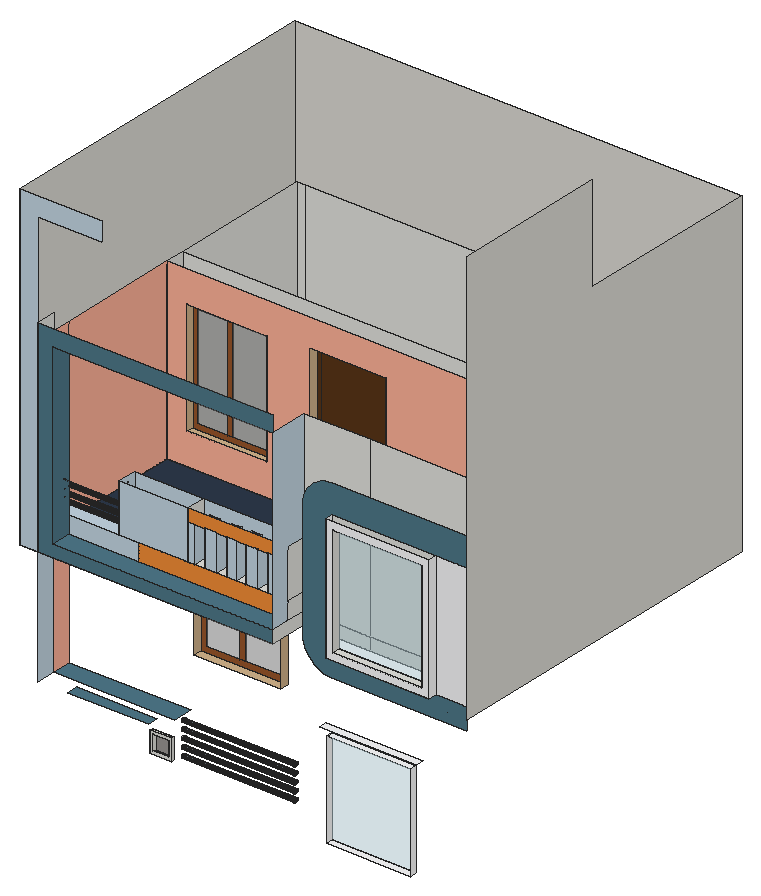
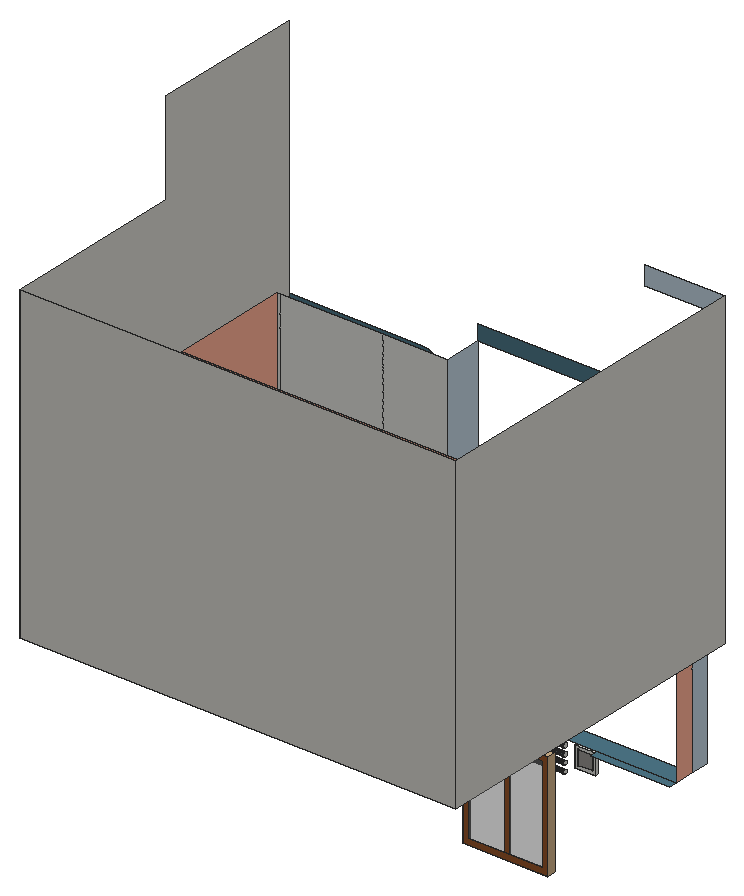
# SketchUp Ruby script. Lengths in inches.
U = 1.inch
M = Sketchup.active_model
def pt(a) = Geom::Point3d.new(a.map { |v| v * U })
def face(e, loops, mat)
  f = e.add_face(loops[0].map { |a| pt(a) })
  loops[1..].each { |l| e.add_face(l.map { |a| pt(a) }).erase! }
  f.material = f.back_material = mat if mat
  f
end
# faces: each face lists its corners as indices into pts; further lists are holes
def faces(e, pts, list, mat = nil) = list.each { |f| face(e, (f[0].is_a?(Array) ? f : [f]).map { |l| l.map { |i| pts[i] } }, mat) }
# xy, xz, yz: faces in a plane at the given z, y or x. An outline is a flat list of corners, or four numbers for a rectangle; further outlines are holes
def ring(l) = l.size == 4 ? [[l[0], l[1]], [l[2], l[1]], [l[2], l[3]], [l[0], l[3]]] : l.each_slice(2).to_a
def flat(e, list, mat, &to3) = list.each { |f| face(e, (f[0].is_a?(Array) ? f : [f]).map { |l| ring(l).map { |u, v| to3.(u, v) } }, mat) }
def xy(e, z, list, mat = nil) = flat(e, list, mat) { |x, y| [x, y, z] }
def xz(e, y, list, mat = nil) = flat(e, list, mat) { |x, z| [x, y, z] }
def yz(e, x, list, mat = nil) = flat(e, list, mat) { |y, z| [x, y, z] }
def lines(e, pts, list) = list.each { |a, b| e.add_line(pt(pts[a]), pt(pts[b])) }
# prism: a flat outline (further loops are holes) pulled along v
def prism(e, loops, v, mat = nil)
  f = face(e, loops, mat); d = Geom::Vector3d.new(v.map { |x| x * U })
  f.pushpull(f.normal.samedirection?(d) ? d.length : -d.length)
end
def box(e, o, s, mat = nil) = prism(e, [[o, [o[0] + s[0], o[1], o[2]], [o[0] + s[0], o[1] + s[1], o[2]], [o[0], o[1] + s[1], o[2]]]], [0, 0, s[2]], mat)
def at(x, y, z, deg = 0) = Geom::Transformation.translation(pt([x, y, z])) * Geom::Transformation.rotation(ORIGIN, Z_AXIS, deg.degrees)
def axes(o, x, y, z) = Geom::Transformation.new([*x, 0, *y, 0, *z, 0, *pt(o).to_a, 1])
def part(name) = M.definitions.add(name)
# library, detail: a bought-in or finely detailed component or shape, given as its bounding box
def library(name, o, s) = part(name).tap { |d| box(d.entities, o, s) }
def detail(e, o, s) = box(e.add_group.entities, o, s)
def put(e, d, t, mat = nil) = e.add_instance(d, t).tap { |i| i.material = mat if mat }
def group(e, t, mat = nil) = e.add_group.tap { |g| g.transformation = t; g.material = mat if mat }.entities
root = M.entities
M.materials.add("[0035_Tan]").color = [210, 180, 140]
M.materials.add("[0096_SkyBlue]").color = [79, 120, 137]
M.materials.add("[Blinds Vertical Pattern]").color = [247, 247, 249]
M.materials.add("[Cladding Siding Tan]").color = [242, 141, 55]
M.materials.add("[Color B02]").color = [255, 178, 153]
M.materials.add("[Concrete Aggregate Smoke]").color = [154, 150, 148]
M.materials.add("[Formica Speckled Grey]").color = [94, 105, 111]
M.materials.add("[Leather Blue]").color = [45, 57, 74]
M.materials.add("[Quartz Light Grey]").color = [251, 251, 252]
M.materials.add("[Terrazzo Light Blue]").color = [196, 214, 227]
M.materials.add("[Terrazzo Tile Light]").color = [219, 217, 210]
M.materials.add("[Translucent Glass Gray]1").color = [128, 128, 128]
M.materials["[Translucent Glass Gray]1"].alpha = 0.5
M.materials.add("[Translucent Glass Safety]").color = [204, 235, 244]
M.materials["[Translucent Glass Safety]"].alpha = 0.5
M.materials.add("[Wood Cherry Original]1").color = [152, 86, 42]
M.materials.add("[Wood Floor Parquet]").color = [89, 54, 24]
xy(root,174.45,[[254.96,158.43,308.4,162.87]],"[Quartz Light Grey]")
xy(root,175.17,[[85.49,265.26,140.61,270.89]],"[0035_Tan]")
xy(root,175.61,[[131.3,173.37,144.73,175.06]])
xy(root,177.5,[[133.18,173.37,142.85,175.06]])
xy(root,187.17,[[133.18,173.37,142.85,175.06]])
xy(root,189.05,[[131.3,173.37,144.73,175.06]])
xy(root,190.75,[[77.92,175.06,129.11,181.62]],"[0096_SkyBlue]")
xy(root,199,[[68.53,175.06,145.53,187.5]],"[0096_SkyBlue]")
xy(root,235.33,[[254.96,158.43,308.4,162.87]],"[Quartz Light Grey]")
xy(root,239.3,[[250.99,158.43,312.37,162.87]],"[Quartz Light Grey]")
xy(root,244.54,[[85.49,265.26,140.61,270.89]],"[0035_Tan]")
xy(root,252.25,[[159.93,265.26,209.68,271.64]],"[0035_Tan]")
xy(root,272.8125,[[57.16,162.87,68.53,175.06],[68.53,265.26,328.05,277.89],[68.53,277.89,73.72,368.29],[73.72,277.89,328.05,368.29]])
xy(root,272.8125,[[68.53,162.87,68.53,265.26,328.05,265.26,328.05,187.5,217.34,187.5,217.34,162.87]],"[Color B02]")
xy(root,280.09,[[254.93,157.81,320.55,162.87]])
xy(root,280.8125,[[68.53,175.18,217.34,187.5],[68.53,265.26,68.53,277.89,328.05,277.89,328.05,265.26,207.48,265.26,207.48,270.7,158.92,270.7,158.92,265.26],[68.53,277.89,328.05,368.29]])
xy(root,280.8125,[[158.92,265.26,207.48,270.7]],"[0035_Tan]")
xy(root,280.8125,[[78.16,162.87,217.34,175.18]],"[0096_SkyBlue]")
xy(root,280.8125,[[68.53,187.5,328.05,265.26]],"[Leather Blue]")
xy(root,284.73,[[259.5625,157.81,315.92,162.87]])
xy(root,291.5625,[[110.1875,175.18,153.69,187.5],[153.69,175.18,158.09,187.5],[158.09,175.18,164.38,187.5],[164.38,175.18,171.84,187.5],[171.84,175.18,178.13,187.5],
  [178.13,175.18,184.46,187.5],[184.46,175.18,190.75,187.5],[190.75,175.18,198.34,187.5],[198.34,175.18,204.63,187.5],[204.63,175.18,217.34,187.5]])
xy(root,291.5625,[[68.53,175.18,110.1875,187.5]],"[Terrazzo Light Blue]")
xy(root,301.03,[[81.24,265.26,131.93,269.39]],"[0035_Tan]")
xz(root,157.81,[[[254.93,280.09,320.55,358.97],[259.5625,284.73,315.92,354.33]]],"[Quartz Light Grey]")
xz(root,162.87,[[[254.93,280.09,320.55,358.97],[259.5625,284.73,315.92,354.33]]])
xz(root,162.87,[[254.82,266.71,340.49,266.71,340.49,280.09,254.93,280.09,254.93,358.97,340.49,358.97,340.49,377.3,254.93,377.3,252.54,377.14,250.18,376.67,247.91,375.9,245.76,374.84,243.77,373.51,241.97,371.93,240.38,370.125,239.05,368.13,237.99,365.98,237.22,363.71,236.75,361.36,236.6,358.97,236.6,284.93,236.75,282.55,237.22,280.21,237.98,277.95,239.04,275.82,240.36,273.84,241.93,272.04,243.72,270.47,245.71,269.15,247.84,268.09,250.1,267.33,252.4375,266.86],[68.53,272.8125,217.34,272.8125,217.34,280.8125,78.16,280.8125,78.16,392.8125,217.34,392.8125,217.34,403.0625,68.53,403.0625]],"[0096_SkyBlue]")
xz(root,162.87,[[320.55,280.09,340.49,358.97]],"[Blinds Vertical Pattern]")
xz(root,162.87,[[57.16,272.8125,68.53,272.8125,68.53,463,109.08,463,109.08,475.0625,57.16,475.0625]],"[Terrazzo Light Blue]")
xz(root,162.87,[[254.96,174.45,308.4,235.33],[259.5625,284.73,315.92,354.33]],"[Translucent Glass Safety]")
xz(root,173.37,[[[131.3,175.61,144.73,189.05],[133.18,177.5,142.85,187.17]]])
xz(root,175.06,[[[131.3,175.61,144.73,189.05],[133.18,177.5,142.85,187.17]]])
xz(root,175.06,[[133.18,177.5,142.85,187.17]],"[Concrete Aggregate Smoke]")
xz(root,175.18,[[68.53,280.8125,78.16,291.5625],[68.53,291.5625,78.16,392.8125]])
xz(root,175.18,[[122.76,280.8125,217.34,291.5625],[210.19,291.5625,217.34,291.5625,217.34,322.125,153.69,322.125,153.69,314.29,210.19,314.29]],"[Cladding Siding Tan]")
xz(root,175.18,[[78.16,280.8125,122.76,291.5625],[110.1875,291.5625,153.69,322.125],[153.69,291.5625,158.09,314.29],[164.38,291.5625,171.84,314.29],[178.13,291.5625,184.46,314.29],
  [190.75,291.5625,198.34,314.29],[204.63,291.5625,210.19,314.29]],"[Terrazzo Light Blue]")
xz(root,187.5,[[217.34,272.8125,259.37,280.8125],[259.37,272.8125,326.14,280.8125],[326.14,272.8125,328.05,280.8125],[217.34,280.8125,259.37,392.8125],[259.37,280.8125,326.14,392.8125],
  [326.14,280.8125,328.05,392.8125]])
xz(root,187.5,[[68.53,280.8125,217.34,291.5625],[110.1875,291.5625,153.69,322.125],[153.69,291.5625,153.69,322.125,217.34,322.125,217.34,291.5625,204.63,291.5625,204.63,314.29,198.34,314.29,198.34,291.5625,190.75,291.5625,190.75,314.29,184.46,314.29,184.46,291.5625,178.13,291.5625,178.13,314.29,171.84,314.29,171.84,291.5625,164.38,291.5625,164.38,314.29,158.09,314.29,158.09,291.5625]],"[Terrazzo Light Blue]")
xz(root,265.26,[[68.53,272.8125,328.05,280.8125]])
xz(root,265.26,[[[68.53,280.8125,158.92,280.8125,158.92,375.1875,207.48,375.1875,207.48,280.8125,328.05,280.8125,328.05,392.8125,68.53,392.8125],[81.24,301.03,131.93,372.97]]],"[Color B02]")
xz(root,269.39,[[84.54,304.33,103.99,369.67],[106.67,304.33,128.62,369.67]],"[Translucent Glass Gray]1")
xz(root,269.39,[[[81.24,301.03,131.93,372.97],[84.54,304.33,128.62,369.67]],[103.99,304.33,106.67,369.67]],"[Wood Cherry Original]1")
xz(root,270.7,[[[158.92,280.8125,207.48,375.1875],[162.2,284.1,204.19,371.9]],[162.2,284.1,204.19,371.9]],"[Wood Floor Parquet]")
xz(root,270.89,[[89.04,178.72,110.22,241],[113.79,178.72,137.07,241]],"[Translucent Glass Gray]1")
xz(root,270.89,[[[85.49,175.17,140.61,244.54],[89.04,178.72,137.07,241]],[110.22,178.72,113.79,241]],"[Wood Cherry Original]1")
xz(root,277.89,[[68.53,272.8125,328.05,280.8125],[68.53,280.8125,328.05,392.8125]])
xz(root,368.29,[[68.53,272.8125,73.72,280.8125],[73.72,272.8125,328.05,280.8125],[68.53,280.8125,73.72,392.8125],[73.72,280.8125,328.05,392.8125]])
xz(root,380.73,[[57.16,272.8125,340.49,475.0625]],"[Terrazzo Tile Light]")
yz(root,57.16,[[162.87,272.8125,380.73,475.0625]],"[Terrazzo Tile Light]")
yz(root,68.53,[[162.87,272.8125,187.5,280.8125],[187.5,272.8125,265.26,280.8125],[265.26,272.8125,277.89,280.8125],[277.89,272.8125,368.29,280.8125],[162.87,280.8125,175.18,403.0625],
  [175.18,280.8125,187.5,291.5625],[265.26,280.8125,277.89,392.8125],[277.89,280.8125,368.29,392.8125]])
yz(root,68.53,[[175.06,199,187.5,272.8125],[187.5,280.8125,265.26,392.8125],[[175.18,291.5625,187.5,392.8125],[181.95,297.93,181.66,297.97,181.39,298.08,181.16,298.26,180.98,298.5,180.86,298.77,180.83,299.06,180.86,299.35,180.98,299.62,181.16,299.85,181.39,300.03,181.66,300.15,181.95,300.18,182.24,300.15,182.51,300.03,182.75,299.85,182.93,299.62,183.04,299.35,183.08,299.06,183.04,298.77,182.93,298.5,182.75,298.26,182.51,298.08,182.24,297.97],[181.95,293.37,181.66,293.41,181.39,293.52,181.16,293.7,180.98,293.93,180.86,294.21,180.83,294.5,180.86,294.79,180.98,295.06,181.16,295.29,181.39,295.47,181.66,295.58,181.95,295.62,182.24,295.58,182.51,295.47,182.75,295.29,182.93,295.06,183.04,294.79,183.08,294.5,183.04,294.21,182.93,293.93,182.75,293.7,182.51,293.52,182.24,293.41],[181.95,303.25,181.66,303.28,181.39,303.4,181.16,303.58,180.98,303.81,180.86,304.08,180.83,304.37,180.86,304.66,180.98,304.93,181.16,305.17,181.39,305.35,181.66,305.46,181.95,305.5,182.24,305.46,182.51,305.35,182.75,305.17,182.93,304.93,183.04,304.66,183.08,304.37,183.04,304.08,182.93,303.81,182.75,303.58,182.51,303.4,182.24,303.28],[181.95,308.5,181.66,308.53,181.39,308.65,181.16,308.83,180.98,309.06,180.86,309.33,180.83,309.62,180.86,309.91,180.98,310.18,181.16,310.42,181.39,310.6,181.66,310.71,181.95,310.75,182.24,310.71,182.51,310.6,182.75,310.42,182.93,310.18,183.04,309.91,183.08,309.62,183.04,309.33,182.93,309.06,182.75,308.83,182.51,308.65,182.24,308.53],[181.95,313,181.66,313.03,181.39,313.15,181.16,313.33,180.98,313.56,180.86,313.83,180.83,314.12,180.86,314.41,180.98,314.68,181.16,314.92,181.39,315.1,181.66,315.21,181.95,315.25,182.24,315.21,182.51,315.1,182.75,314.92,182.93,314.68,183.04,314.41,183.08,314.12,183.04,313.83,182.93,313.56,182.75,313.33,182.51,313.15,182.24,313.03],[181.95,317.18,181.66,317.22,181.39,317.33,181.16,317.51,180.98,317.75,180.86,318.02,180.83,318.31,180.86,318.6,180.98,318.87,181.16,319.1,181.39,319.28,181.66,319.4,181.95,319.43,182.24,319.4,182.51,319.28,182.75,319.1,182.93,318.87,183.04,318.6,183.08,318.31,183.04,318.02,182.93,317.75,182.75,317.51,182.51,317.33,182.24,317.22]]],"[Color B02]")
yz(root,68.53,[[162.87,199,175.06,272.8125]],"[Terrazzo Light Blue]")
yz(root,78.16,[[162.87,280.8125,175.18,392.8125]],"[0096_SkyBlue]")
yz(root,81.24,[[265.26,301.03,269.39,372.97]],"[0035_Tan]")
yz(root,85.49,[[265.26,175.17,270.89,244.54]],"[0035_Tan]")
yz(root,110.1875,[[181.95,293.37,182.24,293.41,182.51,293.52,182.75,293.7,182.93,293.93,183.04,294.21,183.08,294.5,183.04,294.79,182.93,295.06,182.75,295.29,182.51,295.47,182.24,295.58,181.95,295.62,181.66,295.58,181.39,295.47,181.16,295.29,180.98,295.06,180.86,294.79,180.83,294.5,180.86,294.21,180.98,293.93,181.16,293.7,181.39,293.52,181.66,293.41],[181.95,297.93,182.24,297.97,182.51,298.08,182.75,298.26,182.93,298.5,183.04,298.77,183.08,299.06,183.04,299.35,182.93,299.62,182.75,299.85,182.51,300.03,182.24,300.15,181.95,300.18,181.66,300.15,181.39,300.03,181.16,299.85,180.98,299.62,180.86,299.35,180.83,299.06,180.86,298.77,180.98,298.5,181.16,298.26,181.39,298.08,181.66,297.97],[181.95,303.25,182.24,303.28,182.51,303.4,182.75,303.58,182.93,303.81,183.04,304.08,183.08,304.37,183.04,304.66,182.93,304.93,182.75,305.17,182.51,305.35,182.24,305.46,181.95,305.5,181.66,305.46,181.39,305.35,181.16,305.17,180.98,304.93,180.86,304.66,180.83,304.37,180.86,304.08,180.98,303.81,181.16,303.58,181.39,303.4,181.66,303.28]])
yz(root,110.1875,[[[175.18,291.5625,187.5,322.125],[181.95,293.37,182.24,293.41,182.51,293.52,182.75,293.7,182.93,293.93,183.04,294.21,183.08,294.5,183.04,294.79,182.93,295.06,182.75,295.29,182.51,295.47,182.24,295.58,181.95,295.62,181.66,295.58,181.39,295.47,181.16,295.29,180.98,295.06,180.86,294.79,180.83,294.5,180.86,294.21,180.98,293.93,181.16,293.7,181.39,293.52,181.66,293.41],[181.95,313,182.24,313.03,182.51,313.15,182.75,313.33,182.93,313.56,183.04,313.83,183.08,314.12,183.04,314.41,182.93,314.68,182.75,314.92,182.51,315.1,182.24,315.21,181.95,315.25,181.66,315.21,181.39,315.1,181.16,314.92,180.98,314.68,180.86,314.41,180.83,314.12,180.86,313.83,180.98,313.56,181.16,313.33,181.39,313.15,181.66,313.03],[181.95,297.93,182.24,297.97,182.51,298.08,182.75,298.26,182.93,298.5,183.04,298.77,183.08,299.06,183.04,299.35,182.93,299.62,182.75,299.85,182.51,300.03,182.24,300.15,181.95,300.18,181.66,300.15,181.39,300.03,181.16,299.85,180.98,299.62,180.86,299.35,180.83,299.06,180.86,298.77,180.98,298.5,181.16,298.26,181.39,298.08,181.66,297.97],[181.95,308.5,182.24,308.53,182.51,308.65,182.75,308.83,182.93,309.06,183.04,309.33,183.08,309.62,183.04,309.91,182.93,310.18,182.75,310.42,182.51,310.6,182.24,310.71,181.95,310.75,181.66,310.71,181.39,310.6,181.16,310.42,180.98,310.18,180.86,309.91,180.83,309.62,180.86,309.33,180.98,309.06,181.16,308.83,181.39,308.65,181.66,308.53],[181.95,303.25,182.24,303.28,182.51,303.4,182.75,303.58,182.93,303.81,183.04,304.08,183.08,304.37,183.04,304.66,182.93,304.93,182.75,305.17,182.51,305.35,182.24,305.46,181.95,305.5,181.66,305.46,181.39,305.35,181.16,305.17,180.98,304.93,180.86,304.66,180.83,304.37,180.86,304.08,180.98,303.81,181.16,303.58,181.39,303.4,181.66,303.28],[181.95,317.18,182.24,317.22,182.51,317.33,182.75,317.51,182.93,317.75,183.04,318.02,183.08,318.31,183.04,318.6,182.93,318.87,182.75,319.1,182.51,319.28,182.24,319.4,181.95,319.43,181.66,319.4,181.39,319.28,181.16,319.1,180.98,318.87,180.86,318.6,180.83,318.31,180.86,318.02,180.98,317.75,181.16,317.51,181.39,317.33,181.66,317.22]]],"[Terrazzo Light Blue]")
yz(root,131.3,[[173.37,175.61,175.06,189.05]])
yz(root,131.93,[[265.26,301.03,269.39,372.97]],"[0035_Tan]")
yz(root,133.18,[[173.37,177.5,175.06,187.17]])
yz(root,140.61,[[265.26,175.17,270.89,244.54]],"[0035_Tan]")
yz(root,142.85,[[173.37,177.5,175.06,187.17]])
yz(root,144.73,[[173.37,175.61,175.06,189.05]])
yz(root,145.53,[[181.52,174.46,181.21,174.5,180.92,174.62,180.68,174.81,180.49,175.05,180.37,175.34,180.33,175.65,180.37,175.96,180.49,176.24,180.68,176.49,180.92,176.68,181.21,176.8,181.52,176.84,181.82,176.8,182.11,176.68,182.35,176.49,182.54,176.24,182.66,175.96,182.7,175.65,182.66,175.34,182.54,175.05,182.35,174.81,182.11,174.62,181.82,174.5],[181.52,179.59,181.21,179.625,180.92,179.74,180.68,179.93,180.49,180.18,180.37,180.47,180.33,180.77,180.37,181.08,180.49,181.37,180.68,181.61,180.92,181.8,181.21,181.92,181.52,181.96,181.82,181.92,182.11,181.8,182.35,181.61,182.54,181.37,182.66,181.08,182.7,180.77,182.66,180.47,182.54,180.18,182.35,179.93,182.11,179.74,181.82,179.625],[181.52,184.52,181.21,184.5625,180.92,184.68,180.68,184.87,180.49,185.12,180.37,185.4,180.33,185.71,180.37,186.02,180.49,186.3,180.68,186.55,180.92,186.74,181.21,186.86,181.52,186.9,181.82,186.86,182.11,186.74,182.35,186.55,182.54,186.3,182.66,186.02,182.7,185.71,182.66,185.4,182.54,185.12,182.35,184.87,182.11,184.68,181.82,184.5625],[181.52,189.77,181.21,189.8125,180.92,189.93,180.68,190.12,180.49,190.37,180.37,190.65,180.33,190.96,180.37,191.27,180.49,191.55,180.68,191.8,180.92,191.99,181.21,192.11,181.52,192.15,181.82,192.11,182.11,191.99,182.35,191.8,182.54,191.55,182.66,191.27,182.7,190.96,182.66,190.65,182.54,190.37,182.35,190.12,182.11,189.93,181.82,189.8125],[181.52,194.9,181.21,194.9375,180.92,195.06,180.68,195.25,180.49,195.49,180.37,195.78,180.33,196.09,180.37,196.39,180.49,196.68,180.68,196.93,180.92,197.11,181.21,197.23,181.52,197.27,181.82,197.23,182.11,197.11,182.35,196.93,182.54,196.68,182.66,196.39,182.7,196.09,182.66,195.78,182.54,195.49,182.35,195.25,182.11,195.06,181.82,194.9375]])
yz(root,153.69,[[175.18,291.5625,187.5,322.125]])
yz(root,158.09,[[175.18,291.5625,187.5,314.29]],"[Terrazzo Light Blue]")
yz(root,158.92,[[265.26,280.8125,270.7,375.1875]],"[0035_Tan]")
yz(root,164.38,[[175.18,291.5625,187.5,314.29]],"[Terrazzo Light Blue]")
yz(root,171.84,[[175.18,291.5625,187.5,314.29]],"[Terrazzo Light Blue]")
yz(root,178.13,[[175.18,291.5625,187.5,314.29]],"[Terrazzo Light Blue]")
yz(root,184.46,[[175.18,291.5625,187.5,314.29]],"[Terrazzo Light Blue]")
yz(root,190.75,[[175.18,291.5625,187.5,314.29]],"[Terrazzo Light Blue]")
yz(root,198.34,[[175.18,291.5625,187.5,314.29]],"[Terrazzo Light Blue]")
yz(root,204.63,[[175.18,291.5625,187.5,314.29]],"[Terrazzo Light Blue]")
yz(root,207.48,[[265.26,280.8125,270.7,375.1875]],"[0035_Tan]")
yz(root,217.34,[[162.87,272.8125,187.5,280.8125],[175.18,280.8125,187.5,291.5625],[175.18,291.5625,187.5,322.125]])
yz(root,217.34,[[162.87,280.8125,162.87,392.8125,187.5,392.8125,187.5,322.125,175.18,322.125,175.18,280.8125]],"[Terrazzo Light Blue]")
yz(root,254.93,[[157.81,280.09,162.87,358.97]],"[Quartz Light Grey]")
yz(root,254.96,[[158.43,174.45,162.87,235.33]],"[Quartz Light Grey]")
yz(root,259.5625,[[157.81,284.73,162.87,354.33]])
yz(root,308.4,[[158.43,174.45,162.87,235.33]],"[Quartz Light Grey]")
yz(root,315.92,[[157.81,284.73,162.87,354.33]])
yz(root,320.55,[[157.81,280.09,162.87,358.97]],"[Quartz Light Grey]")
yz(root,328.05,[[187.5,272.8125,265.26,280.8125],[265.26,272.8125,277.89,280.8125],[277.89,272.8125,368.29,280.8125],[265.26,280.8125,277.89,392.8125],[277.89,280.8125,368.29,392.8125]])
yz(root,328.05,[[187.5,280.8125,265.26,392.8125]],"[Color B02]")
yz(root,340.49,[[162.87,272.8125,380.73,272.8125,380.73,475.0625,262.25,475.0625,262.25,536.0625,162.87,536.0625]],"[Terrazzo Tile Light]")
p = [[145.53,180.92,174.62],[145.53,181.21,174.5],[217.34,181.21,174.5],[217.34,180.92,174.62],[145.53,181.52,174.46],[217.34,181.52,174.46],
  [145.53,181.82,174.5],[217.34,181.82,174.5],[145.53,182.11,174.62],[217.34,182.11,174.62],[145.53,180.68,174.81],[217.34,180.68,174.81],
  [145.53,182.35,174.81],[217.34,182.35,174.81],[145.53,180.49,175.05],[217.34,180.49,175.05],[145.53,182.54,175.05],[217.34,182.54,175.05],
  [145.53,180.37,175.34],[217.34,180.37,175.34],[145.53,182.66,175.34],[217.34,182.66,175.34],[145.53,180.33,175.65],[217.34,180.33,175.65],
  [145.53,182.7,175.65],[217.34,182.7,175.65],[145.53,180.37,175.96],[217.34,180.37,175.96],[145.53,182.66,175.96],[217.34,182.66,175.96],
  [145.53,180.49,176.24],[217.34,180.49,176.24],[145.53,182.54,176.24],[217.34,182.54,176.24],[145.53,180.68,176.49],[217.34,180.68,176.49],
  [145.53,182.35,176.49],[217.34,182.35,176.49],[145.53,180.92,176.68],[217.34,180.92,176.68],[145.53,182.11,176.68],[217.34,182.11,176.68],
  [145.53,181.21,176.8],[217.34,181.21,176.8],[145.53,181.82,176.8],[217.34,181.82,176.8],[145.53,181.52,176.84],[217.34,181.52,176.84],
  [145.53,180.92,179.74],[145.53,181.21,179.625],[217.34,181.21,179.625],[217.34,180.92,179.74],[145.53,181.52,179.59],[217.34,181.52,179.59],
  [145.53,181.82,179.625],[217.34,181.82,179.625],[145.53,182.11,179.74],[217.34,182.11,179.74],[145.53,180.68,179.93],[217.34,180.68,179.93],
  [145.53,182.35,179.93],[217.34,182.35,179.93],[145.53,180.49,180.18],[217.34,180.49,180.18],[145.53,182.54,180.18],[217.34,182.54,180.18],
  [145.53,180.37,180.47],[217.34,180.37,180.47],[145.53,182.66,180.47],[217.34,182.66,180.47],[145.53,180.33,180.77],[217.34,180.33,180.77],
  [145.53,182.7,180.77],[217.34,182.7,180.77],[145.53,180.37,181.08],[217.34,180.37,181.08],[145.53,182.66,181.08],[217.34,182.66,181.08],
  [145.53,180.49,181.37],[217.34,180.49,181.37],[145.53,182.54,181.37],[217.34,182.54,181.37],[145.53,180.68,181.61],[217.34,180.68,181.61],
  [145.53,182.35,181.61],[217.34,182.35,181.61],[145.53,180.92,181.8],[217.34,180.92,181.8],[145.53,182.11,181.8],[217.34,182.11,181.8],
  [145.53,181.21,181.92],[217.34,181.21,181.92],[145.53,181.82,181.92],[217.34,181.82,181.92],[145.53,181.52,181.96],[217.34,181.52,181.96],
  [145.53,181.21,184.5625],[145.53,181.52,184.52],[217.34,181.52,184.52],[217.34,181.21,184.5625],[145.53,181.82,184.5625],[217.34,181.82,184.5625],
  [145.53,180.92,184.68],[217.34,180.92,184.68],[145.53,182.11,184.68],[217.34,182.11,184.68],[145.53,180.68,184.87],[217.34,180.68,184.87],
  [145.53,182.35,184.87],[217.34,182.35,184.87],[145.53,180.49,185.12],[217.34,180.49,185.12],[145.53,182.54,185.12],[217.34,182.54,185.12],
  [145.53,180.37,185.4],[217.34,180.37,185.4],[145.53,182.66,185.4],[217.34,182.66,185.4],[145.53,180.33,185.71],[217.34,180.33,185.71],
  [145.53,182.7,185.71],[217.34,182.7,185.71],[145.53,180.37,186.02],[217.34,180.37,186.02],[145.53,182.66,186.02],[217.34,182.66,186.02],
  [145.53,180.49,186.3],[217.34,180.49,186.3],[145.53,182.54,186.3],[217.34,182.54,186.3],[145.53,180.68,186.55],[217.34,180.68,186.55],
  [145.53,182.35,186.55],[217.34,182.35,186.55],[145.53,180.92,186.74],[217.34,180.92,186.74],[145.53,182.11,186.74],[217.34,182.11,186.74],
  [145.53,181.21,186.86],[217.34,181.21,186.86],[145.53,181.82,186.86],[217.34,181.82,186.86],[145.53,181.52,186.9],[217.34,181.52,186.9],
  [145.53,180.92,189.93],[145.53,181.21,189.8125],[217.34,181.21,189.8125],[217.34,180.92,189.93],[145.53,181.52,189.77],[217.34,181.52,189.77],
  [145.53,181.82,189.8125],[217.34,181.82,189.8125],[145.53,182.11,189.93],[217.34,182.11,189.93],[145.53,180.68,190.12],[217.34,180.68,190.12],
  [145.53,182.35,190.12],[217.34,182.35,190.12],[145.53,180.49,190.37],[217.34,180.49,190.37],[145.53,182.54,190.37],[217.34,182.54,190.37],
  [145.53,180.37,190.65],[217.34,180.37,190.65],[145.53,182.66,190.65],[217.34,182.66,190.65],[145.53,180.33,190.96],[217.34,180.33,190.96],
  [145.53,182.7,190.96],[217.34,182.7,190.96],[145.53,180.37,191.27],[217.34,180.37,191.27],[145.53,182.66,191.27],[217.34,182.66,191.27],
  [145.53,180.49,191.55],[217.34,180.49,191.55],[145.53,182.54,191.55],[217.34,182.54,191.55],[145.53,180.68,191.8],[217.34,180.68,191.8],
  [145.53,182.35,191.8],[217.34,182.35,191.8],[145.53,180.92,191.99],[217.34,180.92,191.99],[145.53,182.11,191.99],[217.34,182.11,191.99],
  [145.53,181.21,192.11],[217.34,181.21,192.11],[145.53,181.82,192.11],[217.34,181.82,192.11],[145.53,181.52,192.15],[217.34,181.52,192.15],
  [145.53,180.92,195.06],[145.53,181.21,194.9375],[217.34,181.21,194.9375],[217.34,180.92,195.06],[145.53,181.52,194.9],[217.34,181.52,194.9],
  [145.53,181.82,194.9375],[217.34,181.82,194.9375],[145.53,182.11,195.06],[217.34,182.11,195.06],[145.53,180.68,195.25],[217.34,180.68,195.25],
  [145.53,182.35,195.25],[217.34,182.35,195.25],[145.53,180.49,195.49],[217.34,180.49,195.49],[145.53,182.54,195.49],[217.34,182.54,195.49],
  [145.53,180.37,195.78],[217.34,180.37,195.78],[145.53,182.66,195.78],[217.34,182.66,195.78],[145.53,180.33,196.09],[217.34,180.33,196.09],
  [145.53,182.7,196.09],[217.34,182.7,196.09],[145.53,180.37,196.39],[217.34,180.37,196.39],[145.53,182.66,196.39],[217.34,182.66,196.39],
  [145.53,180.49,196.68],[217.34,180.49,196.68],[145.53,182.54,196.68],[217.34,182.54,196.68],[145.53,180.68,196.93],[217.34,180.68,196.93],
  [145.53,182.35,196.93],[217.34,182.35,196.93],[145.53,180.92,197.11],[217.34,180.92,197.11],[145.53,182.11,197.11],[217.34,182.11,197.11],
  [145.53,181.21,197.23],[217.34,181.21,197.23],[145.53,181.82,197.23],[217.34,181.82,197.23],[145.53,181.52,197.27],[217.34,181.52,197.27],
  [110.1875,181.66,293.41],[110.1875,181.39,293.52],[68.53,181.39,293.52],[68.53,181.66,293.41],[110.1875,181.95,293.37],[68.53,181.95,293.37],
  [110.1875,182.24,293.41],[68.53,182.24,293.41],[110.1875,182.51,293.52],[68.53,182.51,293.52],[110.1875,181.16,293.7],[68.53,181.16,293.7],
  [110.1875,182.75,293.7],[68.53,182.75,293.7],[110.1875,180.98,293.93],[68.53,180.98,293.93],[110.1875,182.93,293.93],[68.53,182.93,293.93],
  [110.1875,180.86,294.21],[68.53,180.86,294.21],[110.1875,183.04,294.21],[68.53,183.04,294.21],[110.1875,180.83,294.5],[68.53,180.83,294.5],
  [110.1875,183.08,294.5],[68.53,183.08,294.5],[110.1875,180.86,294.79],[68.53,180.86,294.79],[110.1875,183.04,294.79],[68.53,183.04,294.79],
  [110.1875,180.98,295.06],[68.53,180.98,295.06],[110.1875,182.93,295.06],[68.53,182.93,295.06],[110.1875,181.16,295.29],[68.53,181.16,295.29],
  [110.1875,182.75,295.29],[68.53,182.75,295.29],[110.1875,181.39,295.47],[68.53,181.39,295.47],[110.1875,182.51,295.47],[68.53,182.51,295.47],
  [110.1875,181.66,295.58],[68.53,181.66,295.58],[110.1875,182.24,295.58],[68.53,182.24,295.58],[110.1875,181.95,295.62],[68.53,181.95,295.62],
  [110.1875,181.95,297.93],[110.1875,181.66,297.97],[68.53,181.66,297.97],[68.53,181.95,297.93],[110.1875,182.24,297.97],[68.53,182.24,297.97],
  [110.1875,181.39,298.08],[68.53,181.39,298.08],[110.1875,182.51,298.08],[68.53,182.51,298.08],[110.1875,181.16,298.26],[68.53,181.16,298.26],
  [110.1875,182.75,298.26],[68.53,182.75,298.26],[110.1875,180.98,298.5],[68.53,180.98,298.5],[110.1875,182.93,298.5],[68.53,182.93,298.5],
  [110.1875,180.86,298.77],[68.53,180.86,298.77],[110.1875,183.04,298.77],[68.53,183.04,298.77],[110.1875,180.83,299.06],[68.53,180.83,299.06],
  [110.1875,183.08,299.06],[68.53,183.08,299.06],[110.1875,180.86,299.35],[68.53,180.86,299.35],[110.1875,183.04,299.35],[68.53,183.04,299.35],
  [110.1875,180.98,299.62],[68.53,180.98,299.62],[110.1875,182.93,299.62],[68.53,182.93,299.62],[110.1875,181.16,299.85],[68.53,181.16,299.85],
  [110.1875,182.75,299.85],[68.53,182.75,299.85],[110.1875,181.39,300.03],[68.53,181.39,300.03],[110.1875,182.51,300.03],[68.53,182.51,300.03],
  [110.1875,181.66,300.15],[68.53,181.66,300.15],[110.1875,182.24,300.15],[68.53,182.24,300.15],[110.1875,181.95,300.18],[68.53,181.95,300.18],
  [110.1875,181.95,303.25],[110.1875,181.66,303.28],[68.53,181.66,303.28],[68.53,181.95,303.25],[110.1875,182.24,303.28],[68.53,182.24,303.28],
  [110.1875,181.39,303.4],[68.53,181.39,303.4],[110.1875,182.51,303.4],[68.53,182.51,303.4],[110.1875,181.16,303.58],[68.53,181.16,303.58],
  [110.1875,182.75,303.58],[68.53,182.75,303.58],[110.1875,180.98,303.81],[68.53,180.98,303.81],[110.1875,182.93,303.81],[68.53,182.93,303.81],
  [110.1875,180.86,304.08],[68.53,180.86,304.08],[110.1875,183.04,304.08],[68.53,183.04,304.08],[110.1875,180.83,304.37],[68.53,180.83,304.37],
  [110.1875,183.08,304.37],[68.53,183.08,304.37],[110.1875,180.86,304.66],[68.53,180.86,304.66],[110.1875,183.04,304.66],[68.53,183.04,304.66],
  [110.1875,180.98,304.93],[68.53,180.98,304.93],[110.1875,182.93,304.93],[68.53,182.93,304.93],[110.1875,181.16,305.17],[68.53,181.16,305.17],
  [110.1875,182.75,305.17],[68.53,182.75,305.17],[110.1875,181.39,305.35],[68.53,181.39,305.35],[110.1875,182.51,305.35],[68.53,182.51,305.35],
  [110.1875,181.66,305.46],[68.53,181.66,305.46],[110.1875,182.24,305.46],[68.53,182.24,305.46],[110.1875,181.95,305.5],[68.53,181.95,305.5],
  [328.05,187.5,272.8125],[328.05,162.87,272.8125]]
faces(root,p,[[0,1,2,3],[1,4,5,2],[4,6,7,5],[6,8,9,7],[10,0,3,11],[8,12,13,9],[14,10,11,15],[12,16,17,13],
  [18,14,15,19],[16,20,21,17],[22,18,19,23],[20,24,25,21],[26,22,23,27],[24,28,29,25],[30,26,27,31],[28,32,33,29],
  [34,30,31,35],[32,36,37,33],[38,34,35,39],[36,40,41,37],[42,38,39,43],[40,44,45,41],[46,42,43,47],[44,46,47,45],
  [48,49,50,51],[49,52,53,50],[52,54,55,53],[54,56,57,55],[58,48,51,59],[56,60,61,57],[62,58,59,63],[60,64,65,61],
  [66,62,63,67],[64,68,69,65],[70,66,67,71],[68,72,73,69],[74,70,71,75],[72,76,77,73],[78,74,75,79],[76,80,81,77],
  [82,78,79,83],[80,84,85,81],[86,82,83,87],[84,88,89,85],[90,86,87,91],[88,92,93,89],[94,90,91,95],[92,94,95,93],
  [96,97,98,99],[97,100,101,98],[102,96,99,103],[100,104,105,101],[106,102,103,107],[104,108,109,105],[110,106,107,111],[108,112,113,109],
  [114,110,111,115],[112,116,117,113],[118,114,115,119],[116,120,121,117],[122,118,119,123],[120,124,125,121],[126,122,123,127],[124,128,129,125],
  [130,126,127,131],[128,132,133,129],[134,130,131,135],[132,136,137,133],[138,134,135,139],[136,140,141,137],[142,138,139,143],[140,142,143,141],
  [144,145,146,147],[145,148,149,146],[148,150,151,149],[150,152,153,151],[154,144,147,155],[152,156,157,153],[158,154,155,159],[156,160,161,157],
  [162,158,159,163],[160,164,165,161],[166,162,163,167],[164,168,169,165],[170,166,167,171],[168,172,173,169],[174,170,171,175],[172,176,177,173],
  [178,174,175,179],[176,180,181,177],[182,178,179,183],[180,184,185,181],[186,182,183,187],[184,188,189,185],[190,186,187,191],[188,190,191,189],
  [192,193,194,195],[193,196,197,194],[196,198,199,197],[198,200,201,199],[202,192,195,203],[200,204,205,201],[206,202,203,207],[204,208,209,205],
  [210,206,207,211],[208,212,213,209],[214,210,211,215],[212,216,217,213],[218,214,215,219],[216,220,221,217],[222,218,219,223],[220,224,225,221],
  [226,222,223,227],[224,228,229,225],[230,226,227,231],[228,232,233,229],[234,230,231,235],[232,236,237,233],[238,234,235,239],[236,238,239,237],
  [240,241,242,243],[244,240,243,245],[246,244,245,247],[248,246,247,249],[241,250,251,242],[252,248,249,253],[250,254,255,251],[256,252,253,257],
  [254,258,259,255],[260,256,257,261],[258,262,263,259],[264,260,261,265],[262,266,267,263],[268,264,265,269],[266,270,271,267],[272,268,269,273],
  [270,274,275,271],[276,272,273,277],[274,278,279,275],[280,276,277,281],[278,282,283,279],[284,280,281,285],[282,286,287,283],[286,284,285,287],
  [288,289,290,291],[292,288,291,293],[289,294,295,290],[296,292,293,297],[294,298,299,295],[300,296,297,301],[298,302,303,299],[304,300,301,305],
  [302,306,307,303],[308,304,305,309],[306,310,311,307],[312,308,309,313],[310,314,315,311],[316,312,313,317],[314,318,319,315],[320,316,317,321],
  [318,322,323,319],[324,320,321,325],[322,326,327,323],[328,324,325,329],[326,330,331,327],[332,328,329,333],[330,334,335,331],[334,332,333,335],
  [336,337,338,339],[340,336,339,341],[337,342,343,338],[344,340,341,345],[342,346,347,343],[348,344,345,349],[346,350,351,347],[352,348,349,353],
  [350,354,355,351],[356,352,353,357],[354,358,359,355],[360,356,357,361],[358,362,363,359],[364,360,361,365],[362,366,367,363],[368,364,365,369],
  [366,370,371,367],[372,368,369,373],[370,374,375,371],[376,372,373,377],[374,378,379,375],[380,376,377,381],[378,382,383,379],[382,380,381,383]],"[Formica Speckled Grey]")
lines(root,p,[[384,385]])
